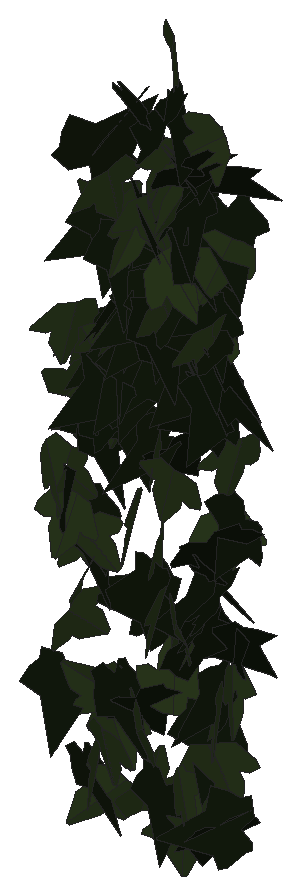
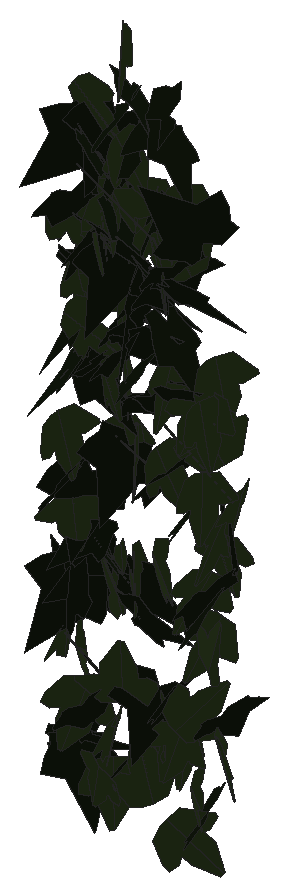
# SketchUp Ruby script. Lengths in inches.
U = 1.inch
M = Sketchup.active_model
def pt(a) = Geom::Point3d.new(a.map { |v| v * U })
def face(e, loops, mat)
  f = e.add_face(loops[0].map { |a| pt(a) })
  loops[1..].each { |l| e.add_face(l.map { |a| pt(a) }).erase! }
  f.material = f.back_material = mat if mat
  f
end
# faces: each face lists its corners as indices into pts; further lists are holes
def faces(e, pts, list, mat = nil) = list.each { |f| face(e, (f[0].is_a?(Array) ? f : [f]).map { |l| l.map { |i| pts[i] } }, mat) }
# xy, xz, yz: faces in a plane at the given z, y or x. An outline is a flat list of corners, or four numbers for a rectangle; further outlines are holes
def ring(l) = l.size == 4 ? [[l[0], l[1]], [l[2], l[1]], [l[2], l[3]], [l[0], l[3]]] : l.each_slice(2).to_a
def flat(e, list, mat, &to3) = list.each { |f| face(e, (f[0].is_a?(Array) ? f : [f]).map { |l| ring(l).map { |u, v| to3.(u, v) } }, mat) }
def xy(e, z, list, mat = nil) = flat(e, list, mat) { |x, y| [x, y, z] }
def xz(e, y, list, mat = nil) = flat(e, list, mat) { |x, z| [x, y, z] }
def yz(e, x, list, mat = nil) = flat(e, list, mat) { |y, z| [x, y, z] }
def lines(e, pts, list) = list.each { |a, b| e.add_line(pt(pts[a]), pt(pts[b])) }
# prism: a flat outline (further loops are holes) pulled along v
def prism(e, loops, v, mat = nil)
  f = face(e, loops, mat); d = Geom::Vector3d.new(v.map { |x| x * U })
  f.pushpull(f.normal.samedirection?(d) ? d.length : -d.length)
end
def box(e, o, s, mat = nil) = prism(e, [[o, [o[0] + s[0], o[1], o[2]], [o[0] + s[0], o[1] + s[1], o[2]], [o[0], o[1] + s[1], o[2]]]], [0, 0, s[2]], mat)
def at(x, y, z, deg = 0) = Geom::Transformation.translation(pt([x, y, z])) * Geom::Transformation.rotation(ORIGIN, Z_AXIS, deg.degrees)
def axes(o, x, y, z) = Geom::Transformation.new([*x, 0, *y, 0, *z, 0, *pt(o).to_a, 1])
def part(name) = M.definitions.add(name)
# library, detail: a bought-in or finely detailed component or shape, given as its bounding box
def library(name, o, s) = part(name).tap { |d| box(d.entities, o, s) }
def detail(e, o, s) = box(e.add_group.entities, o, s)
def put(e, d, t, mat = nil) = e.add_instance(d, t).tap { |i| i.material = mat if mat }
def group(e, t, mat = nil) = e.add_group.tap { |g| g.transformation = t; g.material = mat if mat }.entities
root = M.entities
M.materials.add("efeu1").color = [18, 25, 13]
M.materials.add("efeu2").color = [43, 57, 29]
c1 = part("ivyleaf_10")
p = [[0,0.5,-0.03],[-0.0625,2.02,-0.43],[-0.19,2.01,-0.46],[-0.54,1.05,-0.29],[-0.52,0.625,-0.18],[-0.83,0.76,-0.28],
  [-1.16,0.64,-0.33],[-1.15,0.33,-0.24],[-0.77,-0.39,0.02],[-0.3,-0.51,0.16],[0.04,-0.48,0.23],[-0.02,2.01,-0.4375],
  [-0.06,2.01,-0.43],[0.04,-0.49,0.23],[0.67,-0.49,0.14],[1.38,0.36,-0.2],[1.375,0.51,-0.24],[0.81,0.65,-0.19],
  [0.62,0.59,-0.15],[0.6,1.09,-0.28],[0.5,1.23,-0.31]]
faces(c1.entities,p,[[0,1,2,3,4,5,6,7,8,9,10],[11,12,0,13,14,15,16,17,18,19,20]],"efeu2")
c2 = part("ivyleaf_9")
p = [[1.54,2.16,1.25],[1.36,2.04,1.19],[-0.21,0.99,0.68],[-0.71,1.11,0.82],[-0.85,0.86,0.67],[-0.8,0.17,0.21],
  [-0.9,-0.01,0.1],[-0.67,-0.16,-0.02],[-0.08,-0.08,-0.05],[-0.03,-0.6,-0.4],[0.65,-0.88,-0.66],[0.83,-0.6,-0.49],
  [1.29,-0.42,-0.43],[1.8125,-0.07,-0.26],[1.21,0.44,0.15]]
faces(c2.entities,p,[[0,1,2,3,4,5,6,7,8,9,10,11,12,13,14]],"efeu1")
put(root,c1,axes([576.64,127.54,247.31],[0.70835,-0.80223,-0.06363],[-0.03592,0.05316,-1.07018],[0.80395,0.70922,0.00824]))
put(root,c1,axes([576.73,128.54,258.89],[-0.37335,-0.99679,-0.16906],[0.05103,0.16141,-1.06438],[1.00973,-0.37672,-0.00872]))
put(root,c1,axes([576.76,128.51,261.95],[-0.12433,-1.07799,0.00508],[-0.00296,-0.00478,-1.08514],[1.078,-0.12435,-0.0024]))
put(root,c1,axes([576.59,126.55,257.65],[-0.23742,1.04211,-0.02396],[0.00499,-0.02344,-1.06881],[-1.04237,-0.23747,0.00035]))
put(root,c2,axes([576.32,128.82,254.7],[0.18681,-1.02407,-0.26807],[-0.03313,0.26642,-1.04087],[1.05806,0.18916,0.01474]))
put(root,c1,axes([576.43,128.57,251.5],[-0.1304,-0.28105,-1.01183],[0.24442,-0.99972,0.24619],[-1.0213,-0.20337,0.18811]))
put(root,c2,axes([576.28,127.31,255.46],[-0.06185,0.3458,1.07145],[0.28685,-1.03281,0.34989],[1.08871,0.29177,-0.03132]))
put(root,c1,axes([576.97,127.3,263.26],[-0.40703,-1.02802,0.13133],[-0.02436,-0.13157,-1.10537],[1.03608,-0.40696,0.02561]))
put(root,c1,axes([576.76,127.42,256.55],[0.12929,-0.7996,-0.73511],[0.20649,0.74489,-0.77393],[1.06636,-0.04729,0.23899]))
put(root,c2,axes([576.81,127.23,248.5],[-0.24783,-1.04448,0.09816],[0.00128,-0.10116,-1.0732],[1.04908,-0.24662,0.0245]))
put(root,c1,axes([577.17,126.92,255.6],[1.06841,-0.01307,-0.20658],[-0.20451,0.10109,-1.0641],[0.03196,1.08349,0.09679]))
put(root,c2,axes([576.59,128.67,253.51],[0.43889,-0.90996,0.32836],[0.13148,-0.30112,-1.01021],[0.95842,0.45801,-0.01178]))
put(root,c1,axes([576.87,127.58,260.05],[-0.61465,-0.86358,0.47137],[0.40175,0.28705,1.04975],[-0.89809,0.71944,0.14698]))
put(root,c1,axes([577.15,127.97,262.09],[-0.95876,-0.35925,-0.34635],[0.31121,0.15595,-1.02327],[0.39008,-1.0074,-0.03489]))
put(root,c1,axes([577.9375,128.54,243.6875],[-0.58616,-0.48213,0.86381],[-0.61431,-0.6096,-0.7571],[0.77539,-0.84743,0.05318]))
put(root,c2,axes([576.86,128.14,244.71],[0.64129,-0.82247,-0.0609],[-0.04671,0.0408,-1.04287],[0.8234,0.64288,-0.01172]))
put(root,c2,axes([578.09,128.55,266.97],[-1.07145,0.01709,0.23497],[-0.2355,-0.10751,-1.06606],[0.00642,-1.09163,0.10867]))
put(root,c1,axes([577.29,127.72,254.17],[-0.49189,-0.76298,-0.56099],[0.43837,0.37691,-0.89699],[0.83946,-0.6439,0.13969]))
put(root,c2,axes([577.02,128.6,258.05],[0.50957,-0.93877,-0.00238],[-0.0086,-0.00196,-1.06812],[0.93873,0.50957,-0.0085]))
put(root,c1,axes([578.2,127.74,248.04],[-0.54182,-0.40201,-0.81581],[-0.67266,-0.46199,0.6744],[-0.61211,0.86353,-0.01899]))
put(root,c2,axes([577.21,128.09,269.1875],[-0.25941,-0.18547,1.1415],[1.1159,0.26703,0.29698],[-0.30365,1.13975,0.11618]))
put(root,c1,axes([577.71,126.54,251.6],[-0.30532,-0.73883,-0.79186],[0.26788,0.74564,-0.79899],[1.04936,-0.40532,-0.02644]))
put(root,c1,axes([577.47,128.02,245.23],[0.4628,-0.69474,0.60133],[0.43575,-0.42682,-0.82849],[0.80894,0.62738,0.10226]))
put(root,c2,axes([578.71,127.54,259.78],[-0.87065,0.54795,0.31794],[-0.28012,0.15171,-1.02853],[-0.56822,-0.91438,0.01988]))
put(root,c1,axes([578.32,128.97,259.7],[-0.13333,-1.0273,0.35616],[-0.00822,-0.35787,-1.03529],[1.08726,-0.12868,0.03585]))
put(root,c2,axes([578.74,128.82,262.22],[-0.9675,-0.39914,0.31593],[-0.23955,-0.24168,-1.03894],[0.44915,-0.98867,0.12642]))
put(root,c2,axes([578.98,127.74,264.7],[-0.83934,1.08428,-0.21047],[0.12617,-0.16849,-1.37118],[-1.09729,-0.84876,0.00333]))
put(root,c2,axes([578.375,128.23,267.61],[-0.436,-1.00908,-0.14598],[0.03397,0.1443,-1.09894],[1.01902,-0.43655,-0.02582]))
put(root,c1,axes([578.61,128.16,262.93],[-0.12406,-0.947,-0.52897],[0.10803,0.51899,-0.95446],[1.07933,-0.16079,0.03473]))
put(root,c2,axes([579.21,127.04,261.32],[-1.07287,0.02362,0.17491],[-0.17503,-0.00391,-1.0731],[-0.02268,-1.08703,0.00766]))
put(root,c2,axes([578.18,128.91,259.18],[0.21508,-1.04062,-0.19521],[0.03984,0.20701,-1.05963],[1.05802,0.20375,0.07959]))
put(root,c1,axes([578.47,128.99,255.23],[0.58372,-0.84431,0.41919],[0.25934,-0.33018,-1.02618],[0.90627,0.6383,0.02366]))
put(root,c1,axes([578.22,127.75,267.71],[-0.81451,-0.38997,0.63527],[0.62405,0.1579,0.89705],[-0.40768,1.02081,0.10393]))
put(root,c1,axes([578.61,127.72,247.12],[-0.97308,-0.14751,-0.26125],[0.28207,-0.14773,-0.96721],[0.10221,-0.99665,0.18204]))
put(root,c1,axes([578.9375,126.81,246.78],[-1.00213,0.31844,0.17004],[-0.16221,0.051,-1.05151],[-0.32249,-1.01518,0.00051]))
put(root,c1,axes([579.02,126.8,269.69],[-0.30359,-1.08084,-0.38707],[0.07616,0.38054,-1.12231],[1.14553,-0.31175,-0.02797]))
put(root,c2,axes([579.56,126.95,272.3],[-0.42166,1.02341,0.04885],[-0.01966,0.04474,-1.10688],[-1.02439,-0.42212,0.00114]))
put(root,c2,axes([580.15,128.21,252.07],[-0.54455,0.37526,0.80588],[-0.70043,0.40084,-0.65995],[-0.54742,-0.88618,0.04275]))
put(root,c2,axes([578.92,127.33,249.03],[0.49739,-0.96584,-0.32269],[-0.17141,0.2746,-1.08609],[1.00379,0.52548,-0.02557]))
put(root,c1,axes([579.57,127.76,267.61],[0.61275,-0.85068,-0.41943],[-0.20136,0.37129,-1.04721],[0.92684,0.64307,0.04978]))
put(root,c2,axes([579.12,127.86,266.65],[-0.10616,-1.11959,-0.02287],[-0.02033,0.02489,-1.12438],[1.11964,-0.1057,-0.02258]))
put(root,c2,axes([579.55,128.03,261.79],[-0.72716,-0.78363,0.18193],[0.00731,-0.25166,-1.05477],[0.80443,-0.70606,0.17403]))
put(root,c2,axes([579.65,128.28,261.79],[-0.43095,-1.00679,0.13133],[-0.03914,-0.12609,-1.09506],[1.01456,-0.43251,0.01354]))
put(root,c1,axes([580.44,126.92,247.59],[-0.5977,0.24507,0.94712],[-0.87413,0.36461,-0.64598],[-0.4393,-1.05893,-0.00323]))
put(root,c2,axes([580.22,128.4,264.02],[-0.95637,-0.53642,0.08761],[-0.07808,-0.0399,-1.09653],[0.53789,-0.95954,-0.00339]))
put(root,c2,axes([579.94,127.26,248.54],[0.56739,0.86405,-0.07424],[-0.02965,-0.06934,-1.03361],[-0.86673,0.56801,-0.01324]))
put(root,c2,axes([580.9,127.41,253.0625],[-0.19577,-0.08532,-1.1826],[-1.07073,-0.5021,0.21348],[-0.50927,1.08847,0.00578]))
put(root,c1,axes([580.15,127.15,268.2],[0.28484,0.89749,-0.56787],[-0.38479,-0.46079,-0.92125],[-0.9899,0.43737,0.19471]))
put(root,c2,axes([580.53,128.13,259.06],[-1.05891,0.20526,-0.12121],[0.08461,-0.19235,-1.06487],[-0.22286,-1.04832,0.17166]))
put(root,c1,axes([580.07,128.4,254.58],[0.4828,-0.92419,-0.24784],[0.04829,0.30078,-1.02755],[0.95563,0.45172,0.17714]))
put(root,c2,axes([580.79,128.5625,267.84],[-1.10838,0.10615,0.0495],[-0.04961,0.0012,-1.11344],[-0.10609,-1.10948,0.00353]))
put(root,c1,axes([580.14,127.58,244.375],[-0.30108,-1.12985,0.06045],[0.01569,0.05837,1.16928],[-1.13136,0.30148,0.00013]))
put(root,c2,axes([579.71,128.41,262.96],[0.62604,-0.92533,-0.04327],[0.03837,0.07809,-1.11466],[0.92555,0.62265,0.07548]))
put(root,c2,axes([579.68,127.02,273.18],[0.99649,-0.57605,-0.01614],[0.0367,0.0956,-1.14655],[0.5751,0.99202,0.10113]))
put(root,c2,axes([580.45,126.81,269.05],[0.77696,-0.16809,-0.88948],[-0.83542,0.31824,-0.78988],[0.34858,1.13735,0.08955]))
put(root,c2,axes([580.76,127.62,265.34],[0.27548,-0.14363,-1.1693],[-1.02179,0.56856,-0.31057],[0.58637,1.05825,0.00816]))
put(root,c1,axes([580.61,127.58,259.21],[0.50662,-0.84234,-0.59089],[-0.07944,0.62465,-0.95857],[1.02586,0.46436,0.21758]))
put(root,c2,axes([581.26,127.08,265.3125],[-1.07555,-0.09835,0.22206],[-0.21724,-0.06118,-1.07929],[0.10859,-1.09653,0.0403]))
put(root,c2,axes([580.37,128.85,263.68],[0.15098,-1.08925,-0.05382],[0.00008,0.05434,-1.09964],[1.09058,0.15079,0.00753]))
put(root,c2,axes([581.33,128.07,269.05],[-0.75655,0.80612,-0.11843],[0.0914,-0.07662,-1.10544],[-0.80963,-0.76192,-0.01413]))
put(root,c2,axes([580.91,127.875,258.82],[0.43554,1.00029,0.08354],[0.04101,0.07325,-1.09097],[-1.00293,0.43739,-0.00833]))
put(root,c2,axes([580.57,128.28,264.65],[-0.10441,-1.09457,0.22286],[0.01219,-0.22493,-1.09904],[1.11696,-0.09986,0.03282]))
put(root,c1,axes([580.85,128.25,248.57],[1.14277,0.54693,-0.01227],[-0.00394,0.03665,1.26643],[0.54705,-1.14224,0.03476]))
put(root,c1,axes([580.95,126.78,269.32],[-0.56269,-0.94805,-0.32511],[0.21963,0.24715,-1.10082],[0.97789,-0.60103,0.06016]))
put(root,c1,axes([580.9,127.33,252.89],[0.49609,-0.91619,0.26202],[0.14988,-0.2167,-1.04151],[0.94106,0.51749,0.02775]))
put(root,c2,axes([581.03,128.18,267.05],[0.96993,0.42082,-0.32376],[-0.30982,-0.09898,-1.05683],[-0.43118,1.01774,0.03109]))
put(root,c1,axes([581.48,127.28,262.21],[0.40837,-0.76687,-0.71557],[-0.28997,0.65542,-0.86789],[1.00799,0.49923,0.04023]))
put(root,c1,axes([581.38,128.08,269.27],[-0.76218,-0.8262,0.11751],[0.11826,-0.26448,-1.09243],[0.82609,-0.72442,0.26481]))
put(root,c1,axes([581.42,127.43,271.36],[-0.03194,-1.05145,0.41917],[0.02149,-0.41982,-1.05145],[1.13171,-0.0217,0.03179]))
put(root,c2,axes([582.03,126.18,273.14],[-0.56719,0.89986,0.44017],[-0.26817,0.35098,-1.06306],[-0.96519,-0.62631,0.0367]))
put(root,c1,axes([581.86,127.88,261.83],[0.45422,-0.26332,-1.00179],[-0.63047,0.79762,-0.49551],[0.82184,0.75742,0.17354]))
put(root,c2,axes([582.35,128.05,267.8],[-0.83498,0.51325,0.55525],[-0.5855,0.08455,-0.95862],[-0.47845,-0.99918,0.2041]))
put(root,c1,axes([581.28,128.3,269.01],[-0.77902,0.62595,-0.49887],[0.32596,-0.38771,-0.99549],[-0.73105,-0.8399,0.08774]))
put(root,c2,axes([581.13,127,264.74],[0.2665,-1.08797,-0.04092],[-0.00785,0.04021,-1.12013],[1.08871,0.26661,0.00194]))
put(root,c1,axes([581.64,126.6,265.52],[-0.1134,-1.00262,-0.50322],[0.11405,0.49286,-1.00767],[1.116,-0.15224,0.05185]))
put(root,c2,axes([581.2,127.28,245.31],[0.11623,-1.01794,0.40978],[0.03236,-0.40871,-1.02447],[1.09685,0.11993,-0.0132]))
put(root,c1,axes([581.65,127.09,275.86],[0.76502,-0.75814,-0.39913],[0.0216,0.55198,-1.00707],[0.85652,0.66324,0.38189]))
put(root,c2,axes([582.38,128.27,270.18],[-1.0089,0.46511,0.16794],[-0.18609,-0.00357,-1.10804],[-0.45815,-1.02277,0.08024]))
put(root,c1,axes([582.14,126.6,258.6],[-0.99946,-0.08827,0.40976],[-0.40147,-0.1029,-1.00142],[0.12047,-1.07528,0.06219]))
put(root,c2,axes([581.24,128,270.56],[0.05842,-0.6431,0.92015],[0.53086,-0.79604,-0.59007],[0.98916,0.4652,0.26233]))
put(root,c1,axes([581.53,128.6875,245],[0.87669,-0.21613,0.47187],[0.46856,-0.06876,-0.90204],[0.22321,0.99324,0.04023]))
put(root,c1,axes([581.98,127.99,268.56],[0.59568,-0.95404,-0.14236],[0.03198,0.18676,-1.11776],[0.96407,0.58329,0.12504]))
put(root,c1,axes([582.88,127.37,265.55],[-0.20799,0.00852,-1.15813],[-1.15434,0.09392,0.208],[0.09395,1.1729,-0.00824]))
put(root,c1,axes([581.86,127.72,270.01],[0.00144,-0.4635,1.03889],[0.34441,-0.98996,-0.44215],[1.08421,0.31509,0.13907]))
put(root,c1,axes([582.79,128.46,263.97],[0.41609,-0.07918,-1.10891],[-1.07117,0.28836,-0.42252],[0.29757,1.14876,0.02963]))
put(root,c1,axes([582.23,127.12,244.13],[-0.92004,-0.59382,0.09037],[-0.07593,-0.04901,-1.09504],[0.59584,-0.92317,0.00001]))
put(root,c1,axes([582.64,126.22,252.81],[-0.64511,0.36869,0.73526],[-0.66476,0.31657,-0.74201],[-0.48438,-0.9255,0.03909]))
put(root,c2,axes([581.6875,127.96,272.32],[0.04572,-0.88476,0.68803],[0.15328,-0.6772,-0.88102],[1.11027,0.12992,0.0933]))
put(root,c1,axes([582.17,127.89,267.41],[0.47839,-1.02157,0.13207],[0.04348,-0.12546,-1.12795],[1.02915,0.48016,-0.01374]))
put(root,c2,axes([582.29,128.11,262.16],[-0.56123,-0.72343,0.59695],[-0.11843,-0.63543,-0.88141],[0.93042,-0.51726,0.24788]))
put(root,c2,axes([583.02,127.42,261.66],[0.16875,0.1007,-1.1414],[-1.03053,-0.49106,-0.19568],[-0.50096,1.0441,0.01805]))
put(root,c1,axes([582,126.57,267.18],[0.4675,0.97275,0.52919],[0.23597,0.47371,-1.07924],[-1.08194,0.52364,-0.00672]))
put(root,c1,axes([582.35,126.78,251.5625],[0.74763,-0.76272,0.2847],[-0.16156,0.23986,1.06682],[-0.79793,-0.7632,0.05076]))
put(root,c1,axes([582.31,126.9,246.1],[-0.28884,1.05261,-0.15276],[0.04086,-0.1472,-1.09152],[-1.06285,-0.29171,-0.00044]))
put(root,c2,axes([582.25,128.82,247.73],[-0.23078,-1.0318,0.01328],[-0.01028,-0.01131,-1.05727],[1.03184,-0.23089,-0.00757]))
put(root,c2,axes([582.99,127.74,271.35],[-0.98096,0.50498,-0.31046],[0.24732,-0.19688,-1.1017],[-0.53872,-1.0099,0.05954]))
put(root,c2,axes([583.27,126.61,253.51],[-0.76024,0.62857,0.34419],[-0.25592,0.23056,-0.98634],[-0.66938,-0.80204,-0.0138]))
put(root,c2,axes([582.26,127.25,270.0625],[-0.63967,-0.32249,-0.87641],[0.86919,0.18286,-0.70168],[0.34149,-1.0695,0.1443]))
put(root,c2,axes([582.81,126.26,271.69],[0.50186,0.98803,0.08297],[-0.01361,0.09985,-1.10671],[-0.99142,0.49877,0.05719]))
put(root,c2,axes([582.26,127.88,267.875],[0.51453,-1.14056,-0.41209],[-0.16897,0.37585,-1.25125],[1.20089,0.54157,0.0005]))
put(root,c2,axes([583.22,128.09,249.68],[-0.98629,0.24341,-0.15942],[0.14316,-0.08457,-1.01478],[-0.25332,-0.9955,0.04723]))
put(root,c1,axes([582.82,128.64,255.99],[0.7893,0.73186,-0.06208],[-0.04564,-0.04207,-1.07639],[-0.73307,0.79062,0.00018]))
put(root,c2,axes([582.55,127.32,254.97],[1.04737,-0.14747,-0.01146],[-0.00992,0.01174,-1.05765],[0.14758,1.04736,0.01024]))
put(root,c2,axes([584.02,127.03,265.19],[-0.97407,0.46509,0.56211],[-0.52986,0.19359,-1.07836],[-0.50153,-1.10783,0.04754]))
put(root,c1,axes([583.66,126.92,272.8],[0.70952,-0.23046,-0.83576],[-0.77704,0.30988,-0.74512],[0.38446,1.05161,0.03641]))
put(root,c1,axes([583.38,128.69,259.31],[-0.26439,-1.06404,0.17978],[0.01954,-0.18979,-1.09454],[1.07895,-0.2573,0.06388]))
put(root,c2,axes([583.13,126.1,252.5625],[-0.04082,0.33618,-1.05961],[-0.23301,1.03418,0.33709],[1.08697,0.23432,0.03247]))
put(root,c2,axes([583.72,127.05,244.65],[0.0624,1.0759,-0.27366],[-0.14491,-0.26385,-1.07039],[-1.10066,0.09573,0.12541]))
put(root,c1,axes([583.3,127.57,247.28],[-1.06999,-0.37069,-0.29565],[0.28694,0.07475,-1.13216],[0.37748,-1.10757,0.02255]))
put(root,c2,axes([583.5,126.84,256.34],[0.45507,1.07476,-0.08243],[-0.03762,-0.07358,-1.16712],[-1.07726,0.45658,0.00594]))
put(root,c2,axes([583.02,127.18,265.51],[-0.70866,-0.39424,-0.96987],[0.87424,0.42152,-0.81013],[0.576,-1.1248,0.03634]))
put(root,c1,axes([583.78,127.58,268.07],[-0.79144,-0.64485,0.49543],[-0.21444,-0.50137,-0.99514],[0.78441,-0.78769,0.22782]))
put(root,c2,axes([583.04,128.25,262.15],[0.81458,-0.60055,-0.42224],[-0.24916,0.36711,-1.00282],[0.69056,0.84087,0.13625]))
put(root,c2,axes([583.31,127.68,261.72],[-0.17771,-0.91212,0.58358],[-0.08598,-0.57763,-0.92901],[1.07941,-0.19618,0.02207]))
put(root,c2,axes([582.875,128.56,251.54],[0.04066,-0.17586,1.17807],[0.55763,-1.03879,-0.17432],[1.05253,0.55714,0.04684]))
put(root,c2,axes([584.2,126.51,254.48],[-0.65452,0.806,0.14383],[-0.14811,0.06454,-1.03567],[-0.80523,-0.66702,0.07359]))
put(root,c2,axes([583.28,128.24,269.16],[-0.08333,-1.04976,-0.39497],[0.01673,0.39486,-1.05297],[1.12148,-0.0839,-0.01364]))
put(root,c2,axes([583.25,127.57,263.89],[0.89997,-0.56662,-0.40796],[-0.33401,0.23505,-1.0633],[0.61313,0.95975,0.01956]))
put(root,c1,axes([583.78,126.7,265.04],[-0.29085,-1.14903,-0.25496],[0.0596,0.24791,-1.18527],[1.17547,-0.29688,-0.00299]))
put(root,c2,axes([583.43,127.41,252.19],[0.95596,0.72149,0.12627],[0.10321,0.07285,-1.19766],[-0.72515,0.9615,-0.00401]))
put(root,c2,axes([584.52,127.25,244.82],[-0.75596,-0.04663,0.67598],[-0.65119,-0.22992,-0.7441],[0.18727,-0.98771,0.1413]))
put(root,c2,axes([583.41,127.04,271.18],[0.93297,0.51149,0.33908],[0.24898,0.24845,-1.05986],[-0.56089,0.96109,0.09353]))
put(root,c1,axes([583.36,127.6,249.33],[0.4081,-0.38798,0.93577],[0.68755,-0.63481,-0.56305],[0.74396,0.79951,0.00704]))
put(root,c2,axes([583.64,128.68,256.5],[-0.15103,-0.8563,0.65557],[-0.03694,-0.65747,-0.8673],[1.07781,-0.14253,0.06214]))
put(root,c1,axes([583.73,128.05,250.3],[-0.14793,0.92852,-0.42254],[0.0837,-0.41448,-0.9401],[-1.01671,-0.16922,-0.01592]))
